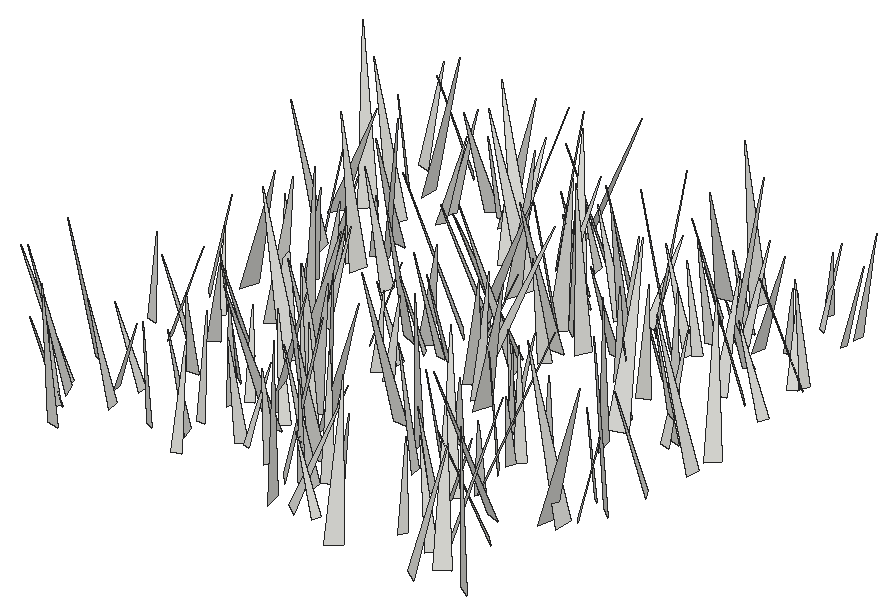
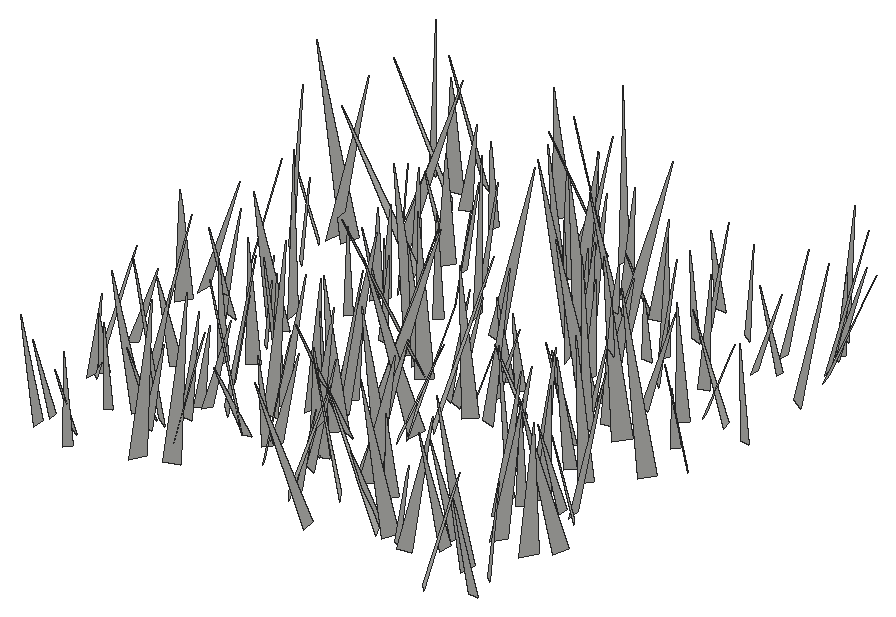
# SketchUp Ruby script. Lengths in inches.
U = 1.inch
M = Sketchup.active_model
def pt(a) = Geom::Point3d.new(a.map { |v| v * U })
def face(e, loops, mat)
  f = e.add_face(loops[0].map { |a| pt(a) })
  loops[1..].each { |l| e.add_face(l.map { |a| pt(a) }).erase! }
  f.material = f.back_material = mat if mat
  f
end
# faces: each face lists its corners as indices into pts; further lists are holes
def faces(e, pts, list, mat = nil) = list.each { |f| face(e, (f[0].is_a?(Array) ? f : [f]).map { |l| l.map { |i| pts[i] } }, mat) }
# xy, xz, yz: faces in a plane at the given z, y or x. An outline is a flat list of corners, or four numbers for a rectangle; further outlines are holes
def ring(l) = l.size == 4 ? [[l[0], l[1]], [l[2], l[1]], [l[2], l[3]], [l[0], l[3]]] : l.each_slice(2).to_a
def flat(e, list, mat, &to3) = list.each { |f| face(e, (f[0].is_a?(Array) ? f : [f]).map { |l| ring(l).map { |u, v| to3.(u, v) } }, mat) }
def xy(e, z, list, mat = nil) = flat(e, list, mat) { |x, y| [x, y, z] }
def xz(e, y, list, mat = nil) = flat(e, list, mat) { |x, z| [x, y, z] }
def yz(e, x, list, mat = nil) = flat(e, list, mat) { |y, z| [x, y, z] }
def lines(e, pts, list) = list.each { |a, b| e.add_line(pt(pts[a]), pt(pts[b])) }
# prism: a flat outline (further loops are holes) pulled along v
def prism(e, loops, v, mat = nil)
  f = face(e, loops, mat); d = Geom::Vector3d.new(v.map { |x| x * U })
  f.pushpull(f.normal.samedirection?(d) ? d.length : -d.length)
end
def box(e, o, s, mat = nil) = prism(e, [[o, [o[0] + s[0], o[1], o[2]], [o[0] + s[0], o[1] + s[1], o[2]], [o[0], o[1] + s[1], o[2]]]], [0, 0, s[2]], mat)
def at(x, y, z, deg = 0) = Geom::Transformation.translation(pt([x, y, z])) * Geom::Transformation.rotation(ORIGIN, Z_AXIS, deg.degrees)
def axes(o, x, y, z) = Geom::Transformation.new([*x, 0, *y, 0, *z, 0, *pt(o).to_a, 1])
def part(name) = M.definitions.add(name)
# library, detail: a bought-in or finely detailed component or shape, given as its bounding box
def library(name, o, s) = part(name).tap { |d| box(d.entities, o, s) }
def detail(e, o, s) = box(e.add_group.entities, o, s)
def put(e, d, t, mat = nil) = e.add_instance(d, t).tap { |i| i.material = mat if mat }
def group(e, t, mat = nil) = e.add_group.tap { |g| g.transformation = t; g.material = mat if mat }.entities
root = M.entities
c1 = part("fur_instance\#9")
p = [[0.8125,0,1.79],[0.67,-0.02,1.48],[0,-0.11,0],[0,0.11,0]]
faces(c1.entities,p,[[0,1,2,3]])
put(root,c1,axes([496.62,198.55,-21.66],[3.4607,5.10853,1.2476],[5.25066,-3.43918,-0.48234],[-0.29016,-1.30574,6.15149]))
put(root,c1,axes([501.49,199.22,-21.66],[-3.98091,-5.38333,3.048],[-6.04161,4.16252,-0.53901],[1.33021,2.79489,6.67363]))
put(root,c1,axes([459,199.9,-21.66],[1.62899,5.48386,2.82302],[6.01922,-2.05055,0.50999],[-1.34582,-2.53344,5.69792]))
put(root,c1,axes([488.71,198.64,-21.66],[-4.66477,5.25581,1.41142],[5.28211,4.8201,-0.49149],[1.30953,-0.72026,7.01013]))
put(root,c1,axes([480.42,201.17,-21.66],[7.19679,1.10507,2.93039],[1.40985,-7.70082,-0.55845],[-2.79655,-1.03845,7.25969]))
put(root,c1,axes([484.96,201.1,-21.66],[-3.33504,1.53851,0.16438],[1.54705,3.32218,0.29368],[0.02564,-0.33558,3.66104]))
put(root,c1,axes([457.33,202.38,-21.66],[2.92591,-1.89098,1.19539],[-1.88086,-3.14489,-0.37117],[-1.21125,0.31559,3.46396]))
put(root,c1,axes([457.41,202.86,-21.66],[-2.05359,-3.75931,0.63579],[-3.81243,2.01617,-0.39286],[-0.04503,0.74602,4.26559]))
put(root,c1,axes([482.45,200.97,-21.66],[3.5807,5.01538,0.32607],[5.01642,-3.54168,-0.61141],[0.30977,-0.61982,6.13202]))
put(root,c1,axes([498,200.85,-21.66],[-2.69969,6.39263,0.77147],[6.43614,2.65406,0.5304],[-0.19237,-0.91623,6.91901]))
put(root,c1,axes([495.49,202.5625,-21.66],[-2.79772,3.91125,0.86225],[4.00509,2.73873,0.57209],[0.02536,-1.03446,4.77471]))
put(root,c1,axes([484.74,204.09,-21.66],[4.77554,-0.30271,1.03368],[-0.19329,-4.86277,-0.53104],[-1.0596,-0.47722,4.75556]))
put(root,c1,axes([469.58,202.46,-21.66],[-0.43977,4.5707,0.64422],[4.59918,0.3789,0.45132],[-0.39225,-0.6818,4.56957]))
put(root,c1,axes([480.7,204.53,-21.66],[-1.22041,-5.00142,1.71972],[-5.19067,1.47111,0.5948],[1.01418,1.51086,5.11369]))
put(root,c1,axes([491.87,203.45,-21.66],[3.56835,-1.26097,2.05366],[-1.59686,-3.9854,0.32755],[-1.80488,1.03305,3.77039]))
put(root,c1,axes([456.5625,204.97,-21.66],[-6.28754,-2.52373,1.27093],[-2.51372,6.41179,0.29625],[1.29062,0.19325,6.76865]))
put(root,c1,axes([481.69,204.93,-21.66],[-6.39617,-0.72322,1.67284],[-0.5993,6.59982,0.56183],[1.72113,-0.38959,6.41236]))
put(root,c1,axes([496.96,202.42,-21.66],[5.77926,4.78065,0.80242],[4.74367,-5.8345,0.5954],[-0.99801,-0.04845,7.47663]))
put(root,c1,axes([460.87,205.18,-21.66],[-4.89796,-0.50596,1.28828],[-0.38248,5.0478,0.52832],[1.33018,-0.4116,4.8956]))
put(root,c1,axes([465.0625,204.67,-21.66],[1.82668,3.73793,1.95155],[3.99067,-2.21946,0.51574],[-1.36206,-1.48974,4.1283]))
put(root,c1,axes([468.2,205.6,-21.66],[-4.55771,-1.35516,1.4154],[-1.26006,4.77117,0.51063],[1.50069,-0.10962,4.72742]))
put(root,c1,axes([476.49,205.8,-21.66],[3.6689,-2.8215,1.45683],[-2.81207,-3.92099,-0.512],[-1.47496,0.45716,4.59995]))
put(root,c1,axes([498.0625,206.8,-21.66],[-4.1053,-4.23157,0.31859],[-4.21802,4.11764,0.33835],[0.46467,-0.00766,5.88602]))
put(root,c1,axes([478.87,204.62,-21.66],[-4.56158,-4.36485,4.54967],[-5.17144,5.80258,0.38189],[3.60662,2.79958,6.30192]))
put(root,c1,axes([455.98,205.95,-21.66],[-6.00367,-1.40851,0.07652],[-1.40991,5.98159,-0.51624],[-0.04369,0.52005,6.14503]))
put(root,c1,axes([472.53,206.98,-21.66],[-2.40754,3.72637,1.88833],[4.14407,2.40561,0.53634],[0.52762,-1.89079,4.40391]))
put(root,c1,axes([482.12,206.08,-21.66],[-1.52023,5.3398,1.43684],[5.52962,1.4775,0.35965],[0.03531,-1.48075,5.54032]))
put(root,c1,axes([479.2,208.52,-21.66],[1.80262,-6.00522,1.15434],[-6.08405,-1.88243,-0.2921],[-0.61598,1.01901,6.26312]))
put(root,c1,axes([459.33,207.67,-21.66],[3.75751,0.05108,0.3502],[0.07903,-3.76142,-0.29936],[-0.34497,-0.30538,3.74592]))
put(root,c1,axes([495.8,209.97,-21.66],[-3.1075,-6.9448,0.74353],[-6.98342,3.07514,-0.46373],[-0.12218,0.86773,7.5942]))
put(root,c1,axes([473.23,206.76,-21.66],[1.4103,3.34023,0.25009],[3.32818,-1.428,0.30438],[-0.37801,-0.11091,3.61295]))
put(root,c1,axes([473.17,210.42,-21.66],[-0.92127,-7.60318,0.93237],[-7.64439,0.85236,-0.60268],[-0.49091,0.99576,7.63504]))
put(root,c1,axes([461.06,208.72,-21.66],[-4.01235,0.08097,0.58825],[0.14386,4.03101,0.42638],[0.5761,-0.44265,3.99045]))
put(root,c1,axes([467.99,207.5625,-21.66],[0.81104,4.54834,1.26147],[4.65262,-0.98593,0.56355],[-0.7949,-1.13006,4.58559]))
put(root,c1,axes([491.64,209.67,-21.66],[3.71055,0.76796,0.33165],[0.80764,-3.68168,-0.51076],[-0.21789,-0.56867,3.7546]))
put(root,c1,axes([455.24,210.58,-21.66],[-3.32824,-5.52708,1.61735],[-5.74671,3.30884,-0.51825],[0.37393,1.65668,6.43096]))
put(root,c1,axes([489.37,210.37,-21.66],[-3.854,-0.48704,1.31581],[-0.33639,4.05498,0.51565],[1.36213,-0.37663,3.85028]))
put(root,c1,axes([468.09,211.41,-21.66],[4.81176,-1.3762,1.70282],[-1.26945,-5.10354,-0.53746],[-1.78382,-0.0803,4.97575]))
put(root,c1,axes([499.65,212.1,-21.66],[8.0282,-2.33719,0.44231],[-2.30718,-8.02996,-0.55383],[-0.57877,-0.40914,8.34313]))
put(root,c1,axes([492.66,212.29,-21.66],[3.43508,-2.31671,0.74566],[-2.27877,-3.51457,-0.42176],[-0.85461,0.05948,4.12177]))
put(root,c1,axes([474.44,213.375,-21.66],[0.33482,-6.22736,0.74708],[-6.26175,-0.28913,0.39628],[0.3585,0.76592,6.22375]))
put(root,c1,axes([471.71,212.11,-21.66],[6.64605,0.23955,0.93352],[0.28653,-6.70181,-0.32012],[-0.92019,-0.35664,6.64266]))
put(root,c1,axes([462.46,213.41,-21.66],[0.91835,-4.65892,0.5996],[-4.68613,-0.86646,0.44487],[0.32448,0.67241,4.72768]))
put(root,c1,axes([486.34,211.91,-21.66],[-5.34365,-1.01248,1.41227],[-1.15776,5.47992,-0.452],[1.29585,0.72082,5.4199]))
put(root,c1,axes([476.36,212.92,-21.66],[7.28234,-1.08518,0.65082],[-1.04869,-7.30325,-0.44316],[-0.70811,-0.34428,7.3494]))
put(root,c1,axes([491.16,210.38,-21.66],[-5.19034,4.80556,0.45379],[4.78626,5.21014,-0.43029],[0.62529,0.00866,7.0603]))
put(root,c1,axes([501.01,212.51,-21.66],[-8.03417,0.61584,1.78735],[0.70083,8.21761,0.3188],[1.75577,-0.4621,8.05143]))
put(root,c1,axes([473.53,211.33,-21.66],[-4.1604,2.35856,0.20079],[2.33408,4.15517,-0.44576],[0.39395,0.28953,4.76162]))
put(root,c1,axes([475.68,212.21,-21.66],[-2.17723,3.86998,1.04919],[4.00343,2.16477,0.32287],[0.22393,-1.07466,4.42864]))
put(root,c1,axes([474.09,214.17,-21.66],[4.71855,-5.46855,1.25045],[-5.59838,-4.69426,0.59612],[-0.35606,1.33873,7.19821]))
put(root,c1,axes([469.01,212.56,-21.66],[-0.87591,3.86506,0.33078],[3.84564,0.82067,0.59405],[-0.50909,-0.4507,3.91829]))
put(root,c1,axes([486.54,215.01,-21.66],[-3.36264,-2.39418,1.21792],[-2.41208,3.55006,0.31902],[1.18208,0.43333,4.11555]))
put(root,c1,axes([492.23,212.94,-21.66],[7.40183,3.33475,0.3809],[3.31775,-7.40888,0.39208],[-0.5081,0.20159,8.10888]))
put(root,c1,axes([466.09,214.87,-21.66],[-3.7574,-4.18768,1.74578],[-4.4509,3.84178,-0.36412],[0.87968,1.55129,5.61445]))
put(root,c1,axes([501.48,213.78,-21.66],[2.95559,2.2846,0.71516],[2.24296,-3.03986,0.44126],[-0.83663,-0.07885,3.70947]))
put(root,c1,axes([484.02,215.43,-21.66],[-6.46976,-1.55499,2.98827],[-1.52534,7.12153,0.40334],[3.00351,0.26714,6.64177]))
put(root,c1,axes([491.48,216.11,-21.66],[-4.27511,-3.26782,2.05551],[-3.38668,4.64678,0.34365],[1.85313,0.95347,5.37002]))
put(root,c1,axes([480.54,217.35,-21.66],[-1.04582,-7.4675,1.55674],[-7.62212,0.96116,-0.50998],[-0.30029,1.61039,7.52311]))
put(root,c1,axes([474,216.46,-21.66],[5.47086,1.91538,2.35531],[2.21322,-5.83902,-0.39241],[-2.07794,-1.17628,5.78316]))
put(root,c1,axes([502.37,216.24,-21.66],[-4.94486,-5.49387,2.91837],[-6.02867,5.15162,-0.51692],[1.53451,2.53562,7.37341]))
put(root,c1,axes([486.1875,217.6,-21.66],[1.68114,-3.92704,0.2758],[-3.91607,-1.63754,0.5539],[0.40264,0.46985,4.23569]))
put(root,c1,axes([459.79,216.66,-21.66],[-3.92921,-1.09616,0.24918],[-1.11465,3.91653,-0.34741],[0.14562,0.40197,4.06442]))
put(root,c1,axes([491.6,217.58,-21.66],[3.2467,-2.02133,0.75684],[-1.94033,-3.33216,-0.57574],[-0.94537,-0.10279,3.78092]))
put(root,c1,axes([457.45,216.84,-21.66],[4.85217,1.44436,0.49792],[1.4914,-4.83766,-0.50049],[-0.33141,-0.62336,5.03778]))
put(root,c1,axes([471.57,217.59,-21.66],[3.82096,-4.05561,2.24215],[-4.19487,-4.26194,-0.56033],[-1.96935,1.20949,5.5438]))
put(root,c1,axes([500.46,217.34,-21.66],[-2.70575,-2.79772,1.42447],[-3.05403,2.78134,-0.3384],[0.7275,1.27058,3.87735]))
put(root,c1,axes([460.53,218.52,-21.66],[2.83156,-3.99697,0.33188],[-4.00855,-2.80696,0.39506],[0.13188,0.49882,4.88236]))
put(root,c1,axes([464.28,218.64,-21.66],[-1.9055,-4.08481,0.78377],[-4.15591,1.83492,-0.5407],[-0.16841,0.93717,4.47485]))
put(root,c1,axes([454.55,218.08,-21.66],[-0.60793,-4.00143,1.69165],[-4.28266,0.83877,0.44495],[0.72934,1.58988,4.02282]))
put(root,c1,axes([470.77,217.58,-21.66],[-4.87312,1.26006,1.29377],[1.19613,5.04128,-0.40455],[1.35309,0.08157,5.01711]))
put(root,c1,axes([492.02,218.22,-21.66],[-4.07522,2.66076,1.05763],[2.66001,4.19896,-0.31421],[1.05952,-0.30776,4.85678]))
put(root,c1,axes([503.12,220.52,-21.66],[-4.38014,-2.49103,0.91186],[-2.44951,4.47381,0.4553],[1.01814,0.04674,5.01832]))
put(root,c1,axes([467.28,219.8,-21.66],[-6.20404,3.776,0.73856],[3.82283,6.20814,0.37243],[0.43544,-0.70326,7.25325]))
put(root,c1,axes([467.59,221.62,-21.66],[6.355,-3.28716,0.66061],[-3.33311,-6.3472,0.48096],[-0.36352,0.73183,7.13864]))
put(root,c1,axes([492.17,221.64,-21.66],[3.31226,-1.52366,0.97308],[-1.49474,-3.45052,-0.31491],[-1.01694,0.10903,3.63228]))
put(root,c1,axes([484.07,223.3,-21.66],[7.12513,-3.29011,0.44393],[-3.26274,-7.13377,-0.50321],[-0.6135,-0.27186,7.83192]))
put(root,c1,axes([487.84,222.25,-21.66],[-1.12295,-3.74744,1.45837],[-3.89173,1.39395,0.58526],[1.01223,1.20198,3.86805]))
put(root,c1,axes([488.26,221.92,-21.66],[2.5994,3.80823,1.24151],[3.99906,-2.55122,-0.54734],[-0.2268,-1.33772,4.57819]))
put(root,c1,axes([475.52,222.0625,-21.66],[-1.6026,3.32948,1.45838],[3.48573,1.8596,-0.41502],[1.03054,-1.11225,3.67172]))
put(root,c1,axes([466.41,223.19,-21.66],[-3.79793,-0.43925,1.06155],[-0.29859,3.91782,0.55288],[1.10936,-0.44932,3.78306]))
put(root,c1,axes([473.73,222.75,-21.66],[-2.42915,2.39744,1.43013],[2.49267,2.71628,-0.31959],[1.25681,-0.75355,3.39799]))
put(root,c1,axes([462.46,223.84,-21.66],[5.72788,-5.11466,1.67521],[-5.30647,-5.77538,0.51083],[-0.89854,1.50329,7.66207]))
put(root,c1,axes([464.77,222.66,-21.66],[1.5886,-5.12639,3.23902],[-5.9044,-2.07062,-0.3813],[-1.38174,2.95423,5.35333]))
put(root,c1,axes([458.28,222.21,-21.66],[-2.65941,2.49787,0.36396],[2.46932,2.68404,-0.37765],[0.52369,0.0288,3.62894]))
put(root,c1,axes([487.35,223.25,-21.66],[0.08392,3.77547,1.67654],[4.10941,-0.2474,0.35143],[-0.42151,-1.66031,3.76001]))
put(root,c1,axes([495.56,224.43,-21.66],[-6.42267,-1.42598,3.31634],[-1.29179,7.22813,0.60623],[3.37087,0.05298,6.55107]))
put(root,c1,axes([481.02,225.87,-21.66],[3.73638,-5.69312,0.32255],[-5.69521,-3.70663,0.54933],[0.28337,0.57053,6.78752]))
put(root,c1,axes([465.59,224.27,-21.66],[-2.07525,-6.86081,3.30693],[-7.48887,2.46229,0.40886],[1.38687,3.02978,7.15613]))
put(root,c1,axes([455.45,224.35,-21.66],[3.51843,3.11531,1.14482],[3.25687,-3.56198,-0.31656],[-0.63919,-1.00114,4.68874]))
put(root,c1,axes([474.41,224.96,-21.66],[-3.5972,0.42819,0.55364],[0.48536,3.61469,0.35791],[0.50428,-0.42464,3.60487]))
put(root,c1,axes([482.87,224.32,-21.66],[4.88657,-1.90502,2.44295],[-2.30886,-5.28158,0.49977],[-2.06549,1.39696,5.22091]))
put(root,c1,axes([457.14,227.28,-21.66],[7.07591,-3.11018,0.05148],[-3.09924,-7.06002,-0.5432],[-0.26559,-0.47663,7.71016]))
put(root,c1,axes([477.3,227.46,-21.66],[-1.94034,-4.30134,0.80925],[-4.30819,2.03312,0.47669],[0.77193,0.53502,4.69459]))
put(root,c1,axes([503.81,225.52,-21.66],[-6.67851,0.63047,0.27765],[0.60623,6.66388,-0.54986],[0.32721,0.52189,6.68563]))
put(root,c1,axes([466.04,225.93,-21.66],[1.29664,4.3065,0.97913],[4.41517,-1.23995,-0.39328],[0.1042,-1.05001,4.48024]))
put(root,c1,axes([476.33,227.68,-21.66],[-1.41742,-4.71426,1.18858],[-4.85717,1.31918,-0.56008],[-0.21176,1.29675,4.89077]))
put(root,c1,axes([470.54,225.98,-21.66],[3.10796,2.24348,0.34109],[2.21254,-3.12436,0.38987],[-0.50422,0.11876,3.81322]))
put(root,c1,axes([472.51,228.41,-21.66],[-2.15861,-6.19615,1.53511],[-6.31129,2.3146,0.46773],[0.95736,1.28794,6.5447]))
put(root,c1,axes([474.16,228.59,-21.66],[4.15858,-4.6502,0.45845],[-4.67236,-4.14601,0.32855],[-0.05962,0.56087,6.22978]))
put(root,c1,axes([474.88,227.47,-21.66],[-3.24657,-1.58505,0.39086],[-1.61743,3.24104,-0.29141],[0.22149,0.43432,3.60107]))
put(root,c1,axes([464.91,227.17,-21.66],[3.97041,-1.42005,1.05601],[-1.57618,-4.01704,0.5243],[-0.80459,0.86179,4.18399]))
put(root,c1,axes([481.81,225.27,-21.66],[4.66085,6.54813,0.11631],[6.5407,-4.64683,-0.4912],[0.3329,-0.37945,8.02249]))
put(root,c1,axes([499.65,228.47,-21.66],[-2.15143,-4.58063,1.63472],[-4.86135,2.07952,-0.57094],[0.14745,1.72526,5.02841]))
put(root,c1,axes([482.51,229.5625,-21.66],[-7.47727,-2.4998,1.10622],[-2.44373,7.5564,0.55783],[1.22512,-0.18436,7.86431]))
put(root,c1,axes([480.77,231.67,-21.66],[-1.44964,-7.72306,0.36058],[-7.72764,1.4358,-0.315],[-0.24346,0.41228,7.85162]))
put(root,c1,axes([499.24,227.625,-21.66],[1.25627,4.75609,0.70963],[4.78282,-1.31187,0.32531],[-0.49861,-0.60066,4.90844]))
put(root,c1,axes([494.11,229.74,-21.66],[-2.25784,-3.06403,1.232],[-3.11024,2.47464,0.4545],[1.1102,0.70132,3.77883]))
put(root,c1,axes([494.85,227.11,-21.66],[-3.53884,7.24303,1.02774],[7.25201,3.62348,-0.56563],[0.96238,-0.67082,8.04145]))
put(root,c1,axes([460.4,231.09,-21.66],[4.90607,-3.46037,0.24315],[-3.44997,-4.91123,-0.28332],[-0.36191,-0.09172,5.99695]))
put(root,c1,axes([503.88,227.96,-21.66],[-5.08982,4.44528,0.70369],[4.40622,5.13821,-0.58816],[0.91699,-0.01575,6.73207]))
put(root,c1,axes([462.67,230.18,-21.66],[2.7967,-3.72992,1.22325],[-3.91864,-2.74089,0.60164],[-0.23004,1.34365,4.62297]))
put(root,c1,axes([475.32,231.88,-21.66],[-6.16047,-5.25921,0.96963],[-5.25018,6.22911,0.42963],[1.01736,0.29959,8.08864]))
put(root,c1,axes([493.21,229.64,-21.66],[3.80415,1.70942,1.42934],[1.7089,-4.05302,0.29902],[-1.42996,-0.29602,4.15984]))
put(root,c1,axes([478.1875,230.34,-21.66],[3.49532,2.40186,0.16337],[2.40303,-3.46356,-0.49202],[0.14512,-0.49771,4.21237]))
put(root,c1,axes([483.39,232.1875,-21.66],[3.00214,-3.52749,1.91618],[-3.65397,-3.39209,-0.51969],[-1.66236,1.08552,4.60282]))
put(root,c1,axes([493.09,232.55,-21.66],[2.23095,-4.80055,1.901],[-5.14348,-2.24733,0.36107],[-0.45138,1.8816,5.28129]))
put(root,c1,axes([482.9,234.16,-21.66],[-0.40917,-7.70862,1.45343],[-7.84037,0.35495,-0.32469],[-0.25296,1.46762,7.71264]))
put(root,c1,axes([476.13,234.24,-21.66],[-4.87517,-3.87645,0.62854],[-3.83008,4.91477,0.6039],[0.86741,-0.08574,6.19915]))
put(root,c1,axes([475.81,233.38,-21.66],[7.43524,-1.67911,0.29476],[-1.69435,-7.42416,0.44731],[-0.18841,0.50147,7.60934]))
put(root,c1,axes([489.75,233.78,-21.66],[4.11916,-1.93041,1.42636],[-1.9279,-4.34864,-0.31782],[-1.42975,0.30221,4.53795]))
put(root,c1,axes([466.17,233.58,-21.66],[-4.97411,1.9133,1.24146],[2.05101,5.05519,0.42681],[0.99764,-0.85328,5.31228]))
put(root,c1,axes([482.89,234.73,-21.66],[-4.49464,-4.79472,1.8462],[-5.03521,4.59856,-0.3156],[1.02201,1.56958,6.56442]))
put(root,c1,axes([495.06,233.97,-21.66],[4.42317,-1.03576,2.17466],[-1.28949,-4.85884,0.30856],[-2.03449,0.82776,4.53233]))
put(root,c1,axes([476.41,235,-21.66],[-4.47388,-2.50611,0.21033],[-2.51468,4.46372,-0.30343],[0.03476,0.36756,5.119]))
put(root,c1,axes([487.04,236.57,-21.66],[-0.08674,-5.50292,0.32115],[-5.49794,0.10952,0.39174],[0.3974,0.31411,5.48965]))
put(root,c1,axes([492.66,235.72,-21.66],[-1.51621,-3.26203,0.55212],[-3.23761,1.58793,0.49084],[0.68086,0.28668,3.56354]))
put(root,c1,axes([462.29,234.77,-21.66],[-6.37075,2.32719,2.17346],[2.54476,6.64308,0.34616],[1.91413,-1.08621,6.77365]))
put(root,c1,axes([457.89,235.78,-21.66],[-6.59248,-1.12335,1.64682],[-1.04061,6.79216,0.46743],[1.70031,-0.1986,6.67115]))
put(root,c1,axes([461.28,235.375,-21.66],[2.88206,-3.90926,2.29022],[-4.22914,-3.29495,-0.30223],[-1.62535,1.64154,4.8474]))
put(root,c1,axes([499.54,237.34,-21.66],[-4.76298,-4.61729,1.21885],[-4.61962,4.89113,0.47635],[1.20999,0.49843,6.61653]))
put(root,c1,axes([502.77,235.8,-21.66],[-3.82314,1.91513,0.41484],[1.95484,3.79049,0.51675],[0.13566,-0.64863,4.24466]))
put(root,c1,axes([462.02,237.27,-21.66],[1.68223,-3.64936,0.16027],[-3.63941,-1.65928,0.41825],[0.31341,0.31999,3.9966]))
put(root,c1,axes([458.8125,235.93,-21.66],[3.85375,-0.57416,0.66525],[-0.65849,-3.86826,0.47595],[-0.58191,0.57487,3.8671]))
put(root,c1,axes([484.83,235.29,-21.66],[-6.58758,2.43197,1.48528],[2.355,6.75255,-0.6115],[1.60454,0.07391,6.99549]))
put(root,c1,axes([486.81,238.22,-21.66],[-0.69172,-7.26259,1.83893],[-7.46362,0.82804,0.46276],[0.64909,1.78171,7.28077]))
put(root,c1,axes([463.13,237.3,-21.66],[6.28919,2.00514,2.27548],[2.25266,-6.59596,-0.4138],[-2.03074,-1.10685,6.58812]))
put(root,c1,axes([480.9,236.9375,-21.66],[4.75602,-4.66812,2.75377],[-5.20371,-4.95731,0.58378],[-1.51526,2.37234,6.63855]))
put(root,c1,axes([457.24,236.52,-21.66],[3.19373,2.97376,0.94617],[2.91746,-3.32577,0.60507],[-1.10768,-0.18543,4.3217]))
put(root,c1,axes([481.98,237.27,-21.66],[3.06348,4.37723,2.06786],[4.6001,-3.39453,0.37061],[-1.50841,-1.46222,5.32989]))
put(root,c1,axes([462.25,239.93,-21.66],[-0.34138,-6.1128,0.75859],[-6.1403,0.39794,0.44341],[0.48829,0.7305,6.10625]))
put(root,c1,axes([497.6,236.69,-21.66],[-1.60174,4.9541,0.61833],[4.97114,1.64265,-0.28364],[0.46172,-0.4996,5.19887]))
put(root,c1,axes([480.11,241.29,-21.66],[0.60186,-6.09784,0.10298],[-6.0697,-0.58883,0.60707],[0.59415,0.16161,6.09732]))
put(root,c1,axes([474.68,238.98,-21.66],[6.67765,-1.57713,2.05629],[-1.75682,-6.93326,0.38749],[-1.90506,0.86558,6.85042]))
put(root,c1,axes([480.15,236.75,-21.66],[2.22729,6.28936,0.04999],[6.2767,-2.22605,0.40869],[-0.40191,0.08939,6.65956]))
put(root,c1,axes([489.95,239.92,-21.66],[4.02018,4.80904,4.066],[5.52928,-5.00439,0.45193],[-3.01434,-2.76593,6.25176]))
put(root,c1,axes([496.625,241.65,-21.66],[1.2889,-4.23263,0.01136],[-4.22076,-1.28617,-0.32791],[-0.31699,-0.08469,4.41236]))
put(root,c1,axes([501.83,241.84,-21.66],[-3.65311,-4.50937,0.62916],[-4.48426,3.70309,0.50402],[0.78847,0.16789,5.78149]))
put(root,c1,axes([454.9375,241.07,-21.66],[5.86888,-2.59714,0.14419],[-2.59865,-5.83866,0.60558],[0.11385,0.61201,6.38922]))
put(root,c1,axes([491.55,240.38,-21.66],[-4.44101,1.77663,0.66677],[1.83519,4.45274,0.3588],[0.48276,-0.58331,4.76973]))
put(root,c1,axes([492.09,240.74,-21.66],[-2.34318,3.21724,1.23905],[3.43189,2.31946,0.46753],[0.3286,-1.2829,3.95253]))
put(root,c1,axes([475.15,240.53,-21.66],[-7.32829,2.58062,0.59876],[2.60966,7.33524,0.32553],[0.45582,-0.50666,7.76257]))
put(root,c1,axes([483.625,241.48,-21.66],[-4.37438,2.14658,0.79892],[2.22863,4.38643,0.41683],[0.52851,-0.72986,4.85482]))
put(root,c1,axes([483.97,242.24,-21.66],[2.50338,-2.82714,1.30611],[-3.05988,-2.54469,0.35667],[-0.57944,1.22368,3.75931]))
put(root,c1,axes([478.91,243.07,-21.66],[-1.67954,-4.60165,1.09216],[-4.72861,1.65608,-0.29411],[0.09072,1.12742,4.88974]))
put(root,c1,axes([491.75,242.79,-21.66],[0.28904,-4.61969,1.68996],[-4.89331,-0.44312,-0.3744],[-0.50298,1.65624,4.61355]))
put(root,c1,axes([501.52,241.09,-21.66],[-2.57238,2.98987,0.10946],[2.97729,2.57237,-0.29516],[0.29502,0.10983,3.93311]))
put(root,c1,axes([502.05,241.97,-21.66],[-4.36363,0.98227,0.81119],[0.91976,4.432,-0.41906],[0.88144,0.23814,4.45315]))
put(root,c1,axes([487.21,241.4375,-21.66],[5.30824,4.83924,1.79848],[4.88732,-5.54151,0.48577],[-1.6634,-0.83881,7.16657]))
put(root,c1,axes([459.97,242.74,-21.66],[-6.35948,3.06032,1.72749],[3.24757,6.48259,0.47123],[1.34279,-1.18457,7.04176]))
put(root,c1,axes([479.55,241.05,-21.66],[-3.35316,6.39569,0.22234],[6.39729,3.34326,0.30873],[-0.17041,-0.34016,7.2148]))
put(root,c1,axes([482.56,244.42,-21.66],[-4.52954,-3.25843,1.35312],[-3.24257,4.71245,0.49358],[1.39071,0.3748,5.55792]))
put(root,c1,axes([495.43,244.32,-21.66],[5.75538,-1.33671,0.29214],[-1.31847,-5.75568,-0.36093],[-0.36579,-0.28603,5.89753]))
put(root,c1,axes([486.23,241.94,-21.66],[-0.08905,4.06249,0.07241],[4.03019,0.09752,-0.5148],[0.51634,-0.06053,4.03072]))
put(root,c1,axes([473.84,241.82,-21.66],[-6.13421,5.52562,0.24546],[5.52788,6.11218,0.5523],[-0.18784,-0.57446,8.23747]))
put(root,c1,axes([470.93,242.63,-21.66],[-3.67286,3.55796,0.5072],[3.52102,3.70767,-0.51167],[0.72023,0.01818,5.08794]))
put(root,c1,axes([456.54,243.13,-21.66],[-6.24341,4.5177,1.05822],[4.50521,6.32678,-0.4296],[1.11019,-0.26807,7.69449]))
put(root,c1,axes([462.73,244.6875,-21.66],[4.30722,-1.10997,0.82887],[-1.21703,-4.32511,0.53238],[-0.66174,0.72977,4.41597]))
put(root,c1,axes([497.57,245.45,-21.66],[0.85171,-3.4207,0.8533],[-3.50883,-0.73716,0.54719],[0.34265,0.95401,3.48241]))
put(root,c1,axes([492.92,244.47,-21.66],[4.37398,5.97616,2.1686],[6.29129,-4.44766,-0.43255],[-0.91492,-2.01317,7.39318]))
put(root,c1,axes([490.18,246.28,-21.66],[-4.23671,-2.59002,0.97553],[-2.55905,4.34534,0.42292],[1.0541,0.13924,4.94763]))
put(root,c1,axes([493.17,246.07,-21.66],[-0.82021,3.34867,1.94688],[3.86928,0.61559,0.57127],[-0.18046,-2.02092,3.4]))
put(root,c1,axes([477.31,246.57,-21.66],[-3.67755,-0.2078,1.11626],[-0.0694,3.8179,0.48208],[1.13331,-0.4405,3.65173]))
put(root,c1,axes([493.97,244.38,-21.66],[0.66695,4.37993,0.08385],[4.36286,-0.67176,0.3871],[-0.39533,-0.02429,4.41347]))
put(root,c1,axes([474.26,245.03,-21.66],[5.20843,4.28763,1.83578],[4.29945,-5.48037,0.60158],[-1.80791,-0.68076,6.71935]))
put(root,c1,axes([462.42,246.44,-21.66],[4.97792,-1.2009,1.19397],[-1.36113,-5.04298,0.6026],[-1.0075,0.87956,5.08515]))
put(root,c1,axes([488.11,249.16,-21.66],[2.21636,-6.61774,0.25451],[-6.61771,-2.20273,0.35418],[0.25535,0.35358,6.97003]))
put(root,c1,axes([464.74,248.74,-21.66],[1.62052,-5.44249,0.65001],[-5.43307,-1.68456,-0.55967],[-0.72449,0.45919,5.65098]))
put(root,c1,axes([477.46,247.57,-21.66],[-4.41159,-3.54695,0.73212],[-3.61607,4.3782,-0.57829],[0.20221,0.91078,5.63104]))
put(root,c1,axes([467.15,247.57,-21.66],[6.16664,-2.56617,1.31423],[-2.70082,-6.22755,0.51287],[-1.00896,0.98602,6.65955]))
put(root,c1,axes([458.95,247.89,-21.66],[7.358,-0.55238,1.16955],[-0.51092,-7.44716,-0.30295],[-1.18825,-0.21839,7.37248]))
put(root,c1,axes([456.65,248.13,-21.66],[-2.76326,-3.0585,1.38467],[-3.15346,2.97986,0.28892],[1.15213,0.82059,4.11176]))
put(root,c1,axes([465.89,248.25,-21.66],[-1.30466,-3.28465,1.2487],[-3.51229,1.2605,-0.354],[0.10971,1.29326,3.5165]))
put(root,c1,axes([469.25,246.54,-21.66],[-0.73079,4.32054,0.1844],[4.30671,0.74406,-0.36572],[0.39156,-0.12013,4.36662]))
put(root,c1,axes([468.4,247.68,-21.66],[5.68273,3.19615,0.64935],[3.24559,-5.67036,-0.49352],[-0.32122,-0.74969,6.50117]))
put(root,c1,axes([500.25,249.15,-21.66],[3.57631,0.31891,0.97988],[0.16002,-3.66803,0.60973],[-1.01797,0.54376,3.53835]))
put(root,c1,axes([490.84,250.16,-21.66],[-6.55699,2.55506,2.62376],[2.8465,6.94107,0.35432],[2.30431,-1.30376,7.02829]))
put(root,c1,axes([473.3,250.29,-21.66],[6.47298,0.85818,0.33872],[0.84258,-6.4766,0.30739],[-0.37587,0.26066,6.52238]))
put(root,c1,axes([459.87,252.45,-21.66],[-3.79874,-3.55526,0.6962],[-3.51199,3.8615,0.55657],[0.88909,0.06302,5.17306]))
put(root,c1,axes([500.41,250.86,-21.66],[4.80103,-0.44543,1.50068],[-0.59366,-4.99749,0.41591],[-1.44845,0.57184,4.80368]))
put(root,c1,axes([496.32,252.24,-21.66],[3.38817,-1.89067,0.4047],[-1.85762,-3.4096,-0.37677],[-0.53632,-0.13453,3.86165]))
put(root,c1,axes([497.3,250.08,-21.66],[1.47589,3.3854,0.35503],[3.34161,-1.51469,0.55196],[-0.64858,-0.1002,3.65165]))
put(root,c1,axes([455.94,250.95,-21.66],[0.58745,4.61701,1.14714],[4.75417,-0.52722,-0.31264],[0.17496,-1.17604,4.64372]))
